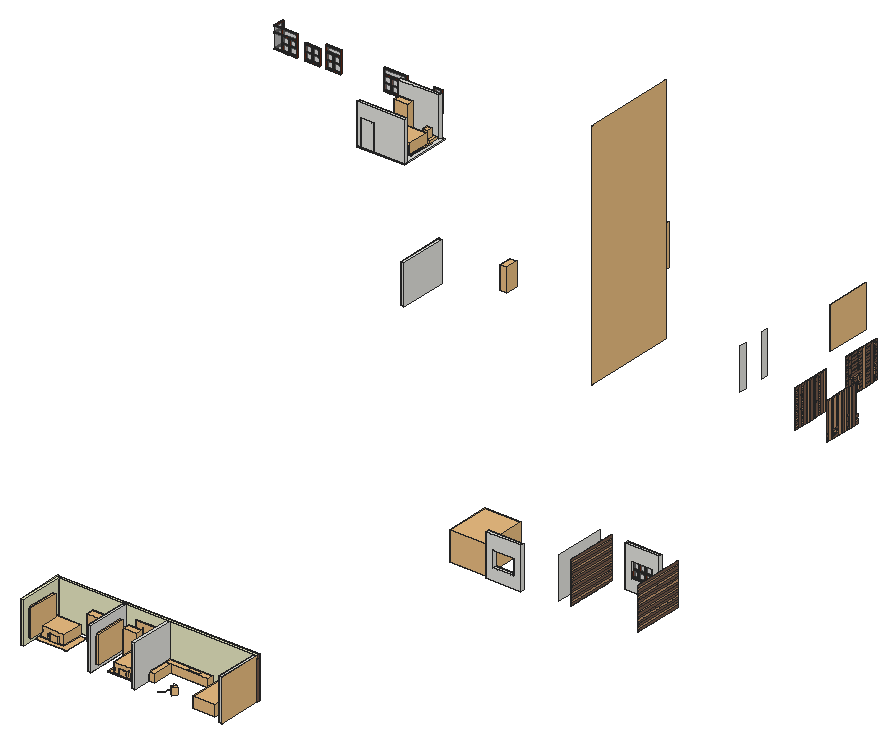
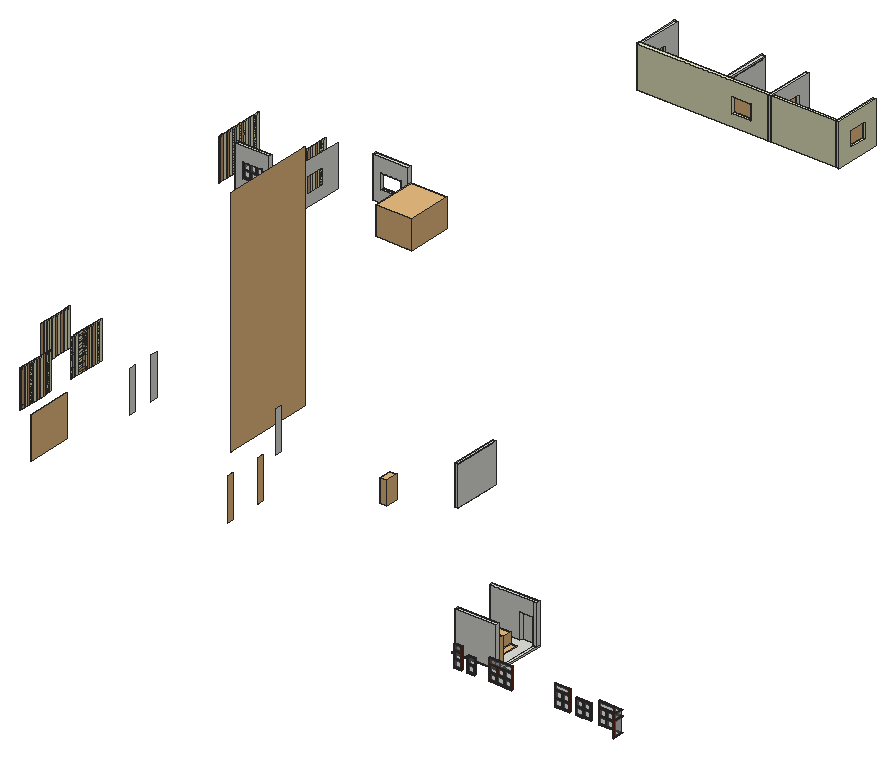
# SketchUp Ruby script. Lengths in inches.
U = 1.inch
M = Sketchup.active_model
def pt(a) = Geom::Point3d.new(a.map { |v| v * U })
def face(e, loops, mat)
  f = e.add_face(loops[0].map { |a| pt(a) })
  loops[1..].each { |l| e.add_face(l.map { |a| pt(a) }).erase! }
  f.material = f.back_material = mat if mat
  f
end
# faces: each face lists its corners as indices into pts; further lists are holes
def faces(e, pts, list, mat = nil) = list.each { |f| face(e, (f[0].is_a?(Array) ? f : [f]).map { |l| l.map { |i| pts[i] } }, mat) }
# xy, xz, yz: faces in a plane at the given z, y or x. An outline is a flat list of corners, or four numbers for a rectangle; further outlines are holes
def ring(l) = l.size == 4 ? [[l[0], l[1]], [l[2], l[1]], [l[2], l[3]], [l[0], l[3]]] : l.each_slice(2).to_a
def flat(e, list, mat, &to3) = list.each { |f| face(e, (f[0].is_a?(Array) ? f : [f]).map { |l| ring(l).map { |u, v| to3.(u, v) } }, mat) }
def xy(e, z, list, mat = nil) = flat(e, list, mat) { |x, y| [x, y, z] }
def xz(e, y, list, mat = nil) = flat(e, list, mat) { |x, z| [x, y, z] }
def yz(e, x, list, mat = nil) = flat(e, list, mat) { |y, z| [x, y, z] }
def lines(e, pts, list) = list.each { |a, b| e.add_line(pt(pts[a]), pt(pts[b])) }
# prism: a flat outline (further loops are holes) pulled along v
def prism(e, loops, v, mat = nil)
  f = face(e, loops, mat); d = Geom::Vector3d.new(v.map { |x| x * U })
  f.pushpull(f.normal.samedirection?(d) ? d.length : -d.length)
end
def box(e, o, s, mat = nil) = prism(e, [[o, [o[0] + s[0], o[1], o[2]], [o[0] + s[0], o[1] + s[1], o[2]], [o[0], o[1] + s[1], o[2]]]], [0, 0, s[2]], mat)
def at(x, y, z, deg = 0) = Geom::Transformation.translation(pt([x, y, z])) * Geom::Transformation.rotation(ORIGIN, Z_AXIS, deg.degrees)
def axes(o, x, y, z) = Geom::Transformation.new([*x, 0, *y, 0, *z, 0, *pt(o).to_a, 1])
def part(name) = M.definitions.add(name)
# library, detail: a bought-in or finely detailed component or shape, given as its bounding box
def library(name, o, s) = part(name).tap { |d| box(d.entities, o, s) }
def detail(e, o, s) = box(e.add_group.entities, o, s)
def put(e, d, t, mat = nil) = e.add_instance(d, t).tap { |i| i.material = mat if mat }
def group(e, t, mat = nil) = e.add_group.tap { |g| g.transformation = t; g.material = mat if mat }.entities
root = M.entities
M.materials.add("02 - Default1").color = [198, 154, 113]
M.materials.add("1").color = [234, 234, 196]
M.materials.add("3").color = [118, 89, 74]
M.materials.add("Material1 metal").color = [192, 192, 192]
M.materials.add("[Color_B17]").color = [102, 40, 20]
M.materials.add("[Translucent_Glass_Gray]").color = [128, 128, 128]
M.materials["[Translucent_Glass_Gray]"].alpha = 0.5
M.materials.add("putih ceramic").color = [255, 255, 255]
c1 = library("HMI+SHE+SAID+BARSTOOL",[-9.1,-9.7,0],[19.23,19.64,34.25])
c2 = part("Component\#33")
prism(c2.entities,[[[0.91,0.01,0.74],[0.87,0.05,0.89],[0.79,0.11,1.01],[0.7,0.18,1.1],[0.58,0.27,1.16],[0.46,0.36,1.18],[0.34,0.46,1.16],[0.23,0.55,1.1],[0.14,0.62,1.01],[0.0625,0.68,0.89],[0.02,0.72,0.74],[0,0.73,0.59],[0.02,0.72,0.4375],[0.0625,0.68,0.3],[0.14,0.62,0.17],[0.23,0.55,0.08],[0.34,0.46,0.02],[0.46,0.36,0],[0.58,0.27,0.02],[0.7,0.18,0.08],[0.79,0.11,0.17],[0.87,0.05,0.3],[0.91,0.01,0.4375],[0.93,0,0.59]]],[0.12,0.15,0],"Material1 metal")
c3 = library("Group10",[-94.75,-3.97,0],[199.87,106.11,39.4375])
c4 = library("mesh-258",[-96.03,-121.28,21.97],[201.42,163.89,40.48])
c5 = library("Group14",[-46.92,-34.29,0],[94.87,68.58,31.875])
c6 = library("Group16",[-47.82,-34.55,0],[96.75,69.58,33.34])
c7 = library("Group18",[-33.62,-26.58,0],[67.24,53.16,20.44])
c8 = library("Group20",[-0.01,-0.01,0.02],[107.76,124.16,6.31])
c9 = library("mesh-263",[-97.08,-118.58,12.75],[201.41,233.93,94.93])
c10 = library("mesh-264",[-106.11,-80.86,12.52],[217.88,74.95,54.44])
c11 = part("Group9")
put(c11.entities,c3,axes([-2.83,3.64,23.125],[0.96274,0,0],[0,0.96274,0],[0,0,0.96274]))
g1 = group(c11.entities,at(-2.83,3.64,23.41))
put(g1,c4,axes([0,0,-21.09],[0.96274,0,0],[0,0.96274,0],[0,0,0.96274]))
put(c11.entities,c5,at(49.15,58.47,50.125))
put(c11.entities,c6,at(-47.3,60.89,49.06))
put(c11.entities,c7,at(-22.74,14.21,61.08))
put(c11.entities,c8,axes([-96.54,-113.26,0],[1.80992,0,0],[0,1.80992,0],[0,0,1.80992]))
g2 = group(c11.entities,at(-2.83,1.61,11.33))
put(g2,c9,at(0,0,-12.75))
g3 = group(c11.entities,at(-2.83,20.36,11.1))
put(g3,c10,at(0,0,-12.52))
c12 = library("Window curtains 2",[0,-81.89,0],[92,82.37,8.12])
c13 = library("Group\#201",[0,0,0],[0.82,117.2,114.11])
c14 = library("mesh-256",[-120.04,-169.59,0.14],[253.19,307.8,1.7])
c15 = part("Group7")
put(c15.entities,c14,at(0,0,0))
c16 = library("COMEDOR+3",[0,0,-3.47],[105.08,67.9,32.46])
c17 = library("Kitchen base cabinets \#1",[0,0,0],[91.73,24.71,35.43])
c18 = library("Group26",[-8.72,-28.73,0.18],[47.65,50.07,77.26])
c19 = library("Group",[-44.49,-44.49,0],[88.98,89.04,25.37])
c20 = library("Dressing_table",[0,-6.3125,-0.01],[54.59,27.125,100.87])
c21 = library("Kitchen base cabinets",[0,0,0],[24.71,188.98,35.43])
c22 = library("coz_ll_125-50",[0,0,0],[49.21,19.69,5.91])
c23 = part("Group\#331")
xy(c23.entities,0,[[0,0,0.82,6.2]],"1")
xy(c23.entities,114.11,[[0,0,0.82,6.2]],"1")
xz(c23.entities,0,[[0,0,0.82,114.11]],"1")
xz(c23.entities,6.2,[[0,0,0.82,114.11]],"1")
yz(c23.entities,0,[[0,0,6.2,114.11]],"1")
yz(c23.entities,0.82,[[0,0,6.2,114.11]],"3")
c24 = part("Group\#330")
put(c24.entities,c23,axes([-0.82,0,0],[1,0,0],[0,1.45243,0],[0,0,1]),"1")
c25 = part("Group\#329")
box(c25.entities,[0,0,0],[0.82,6.2,114.11],"02 - Default1")
c26 = part("Group\#328")
put(c26.entities,c25,axes([-0.82,0,0],[1,0,0],[0,1.45243,0],[0,0,1]))
c27 = part("Group\#286")
put(c27.entities,c24,axes([0.82,0,0],[1,0,0],[0,0.6885,0],[0,0,1]),"02 - Default1")
put(c27.entities,c24,axes([0.82,6.2,89.22],[1,0,0],[0,0,0.67033],[0,-0.05434,0]),"02 - Default1")
put(c27.entities,c24,axes([0.82,6.2,12.68],[1,0,0],[0,0,0.67033],[0,-0.05434,0]),"02 - Default1")
put(c27.entities,c26,axes([0.82,6.2,63.7],[1,0,0],[0,0,0.67033],[0,-0.05434,0]),"02 - Default1")
put(c27.entities,c26,axes([0.82,6.2,25.75],[1,0,0],[0,0,0.67033],[0,-0.05434,0]),"02 - Default1")
put(c27.entities,c26,axes([0.82,6.2,82.99],[1,0,0],[0,0,0.67033],[0,-0.05434,0]),"02 - Default1")
put(c27.entities,c24,axes([0.82,6.2,50.83],[1,0,0],[0,0,0.67033],[0,-0.05434,0]),"02 - Default1")
put(c27.entities,c24,axes([0.82,6.2,76.54],[1,0,0],[0,0,0.67033],[0,-0.05434,0]),"02 - Default1")
put(c27.entities,c24,axes([0.82,6.2,31.98],[1,0,0],[0,0,0.67033],[0,-0.05434,0]),"02 - Default1")
put(c27.entities,c26,axes([0.82,6.2,44.6],[1,0,0],[0,0,0.67033],[0,-0.05434,0]),"02 - Default1")
g4 = group(c27.entities,at(0.82,6.2,95.39),"02 - Default1")
put(g4,c23,axes([-0.82,0,0],[1,0,0],[0,0,0.97361],[0,-0.05434,0]),"1")
put(c27.entities,c26,axes([0.82,6.2,101.84],[1,0,0],[0,0,0.67033],[0,-0.05434,0]),"02 - Default1")
put(c27.entities,c24,axes([0.82,6.2,0],[1,0,0],[0,0,0.67033],[0,-0.05434,0]),"02 - Default1")
put(c27.entities,c24,axes([0.82,6.2,19.3],[1,0,0],[0,0,0.67033],[0,-0.05434,0]),"02 - Default1")
put(c27.entities,c24,axes([0.82,6.2,69.93],[1,0,0],[0,0,0.67033],[0,-0.05434,0]),"02 - Default1")
put(c27.entities,c26,axes([0.82,6.2,6.45],[1,0,0],[0,0,0.67033],[0,-0.05434,0]),"02 - Default1")
put(c27.entities,c24,axes([0.82,6.2,38.15],[1,0,0],[0,0,0.67033],[0,-0.05434,0]),"02 - Default1")
put(c27.entities,c24,axes([0.82,6.2,57.25],[1,0,0],[0,0,0.67033],[0,-0.05434,0]),"02 - Default1")
put(c27.entities,c24,axes([0.82,6.2,108.07],[1,0,0],[0,0,0.67033],[0,-0.05434,0]),"02 - Default1")
c28 = library("kitchen mas haris",[0,0,0],[110.24,135.43,86.61])
c29 = part("Group\#244")
put(c29.entities,c24,axes([0.82,0,0],[1,0,0],[0,0.6885,0],[0,0,1]),"02 - Default1")
put(c29.entities,c26,axes([0.82,6.625,0],[1,0,0],[0,0.6885,0],[0,0,1]),"02 - Default1")
put(c29.entities,c26,axes([0.82,26.45,0],[1,0,0],[0,0.6885,0],[0,0,1]),"02 - Default1")
put(c29.entities,c24,axes([0.82,13.03,0],[1,0,0],[0,0.6885,0],[0,0,1]),"02 - Default1")
put(c29.entities,c24,axes([0.82,32.84,0],[1,0,0],[0,0.6885,0],[0,0,1]),"02 - Default1")
put(c29.entities,c24,axes([0.82,19.82,0],[1,0,0],[0,0.6885,0],[0,0,1]),"02 - Default1")
g5 = group(c29.entities,at(0,117.2,0))
put(g5,c24,axes([0.82,0,0],[1,0,0],[0,0,0.67033],[0,-1.0271,0]),"02 - Default1")
put(g5,c26,axes([0.82,0,101.84],[1,0,0],[0,0,0.67033],[0,-1.0271,0]),"02 - Default1")
put(g5,c26,axes([0.82,0,6.45],[1,0,0],[0,0,0.67033],[0,-1.0271,0]),"02 - Default1")
put(g5,c24,axes([0.82,0,69.93],[1,0,0],[0,0,0.67033],[0,-1.0271,0]),"02 - Default1")
put(g5,c24,axes([0.82,0,95.39],[1,0,0],[0,0,0.67033],[0,-1.0271,0]),"02 - Default1")
put(g5,c24,axes([0.82,0,38.15],[1,0,0],[0,0,0.67033],[0,-1.0271,0]),"02 - Default1")
put(g5,c26,axes([0.82,0,25.75],[1,0,0],[0,0,0.67033],[0,-1.0271,0]),"02 - Default1")
put(g5,c24,axes([0.82,0,31.98],[1,0,0],[0,0,0.67033],[0,-1.0271,0]),"02 - Default1")
put(g5,c24,axes([0.82,0,50.83],[1,0,0],[0,0,0.67033],[0,-1.0271,0]),"02 - Default1")
put(g5,c24,axes([0.82,0,108.07],[1,0,0],[0,0,0.67033],[0,-1.0271,0]),"02 - Default1")
put(g5,c24,axes([0.82,0,89.22],[1,0,0],[0,0,0.67033],[0,-1.0271,0]),"02 - Default1")
put(g5,c24,axes([0.82,0,57.25],[1,0,0],[0,0,0.67033],[0,-1.0271,0]),"02 - Default1")
put(g5,c26,axes([0.82,0,63.7],[1,0,0],[0,0,0.67033],[0,-1.0271,0]),"02 - Default1")
put(g5,c24,axes([0.82,0,12.68],[1,0,0],[0,0,0.67033],[0,-1.0271,0]),"02 - Default1")
put(g5,c26,axes([0.82,0,44.6],[1,0,0],[0,0,0.67033],[0,-1.0271,0]),"02 - Default1")
put(g5,c24,axes([0.82,0,76.54],[1,0,0],[0,0,0.67033],[0,-1.0271,0]),"02 - Default1")
put(g5,c24,axes([0.82,0,19.3],[1,0,0],[0,0,0.67033],[0,-1.0271,0]),"02 - Default1")
put(g5,c26,axes([0.82,0,82.99],[1,0,0],[0,0,0.67033],[0,-1.0271,0]),"02 - Default1")
put(c29.entities,c26,axes([0.82,45.81,0],[1,0,0],[0,0.6885,0],[0,0,1]),"02 - Default1")
put(c29.entities,c24,axes([0.82,52.21,0],[1,0,0],[0,0.6885,0],[0,0,1]),"02 - Default1")
put(c29.entities,c24,axes([0.82,39.18,0],[1,0,0],[0,0.6885,0],[0,0,1]),"02 - Default1")
put(c29.entities,c26,axes([0.82,85.24,0],[1,0,0],[0,0.6885,0],[0,0,1]),"02 - Default1")
put(c29.entities,c24,axes([0.82,78.62,0],[1,0,0],[0,0.6885,0],[0,0,1]),"02 - Default1")
put(c29.entities,c24,axes([0.82,58.8,0],[1,0,0],[0,0.6885,0],[0,0,1]),"02 - Default1")
put(c29.entities,c26,axes([0.82,65.42,0],[1,0,0],[0,0.6885,0],[0,0,1]),"02 - Default1")
put(c29.entities,c24,axes([0.82,71.82,0],[1,0,0],[0,0.6885,0],[0,0,1]),"02 - Default1")
put(c29.entities,c24,axes([0.82,91.64,0],[1,0,0],[0,0.6885,0],[0,0,1]),"02 - Default1")
put(c29.entities,c26,axes([0.82,104.6,0],[1,0,0],[0,0.6885,0],[0,0,1]),"02 - Default1")
put(c29.entities,c24,axes([0.82,111,0],[1,0,0],[0,0.6885,0],[0,0,1]),"02 - Default1")
put(c29.entities,c24,axes([0.82,97.98,0],[1,0,0],[0,0.6885,0],[0,0,1]),"02 - Default1")
c30 = part("Framed panel")
g6 = group(c30.entities,at(0,0,0))
prism(g6,[[[0,22.64,0],[21.26,22.64,0],[21.26,0,0],[0,0,0]],[[1.57,1.57,0],[19.69,1.57,0],[19.69,21.0625,0],[1.57,21.0625,0]]],[0,0,1.57],"[Color_B17]")
g7 = group(c30.entities,at(1.57,1.57,1.02))
xy(g7,0,[[0,0,18.11,19.49]],"[Translucent_Glass_Gray]")
c31 = part("Group\#25")
put(c31.entities,c30,at(0,21.0625,1.57))
put(c31.entities,c30,at(0,0,0))
c32 = part("Group\#47")
g8 = group(c32.entities,at(0,0,0))
prism(g8,[[[70.87,0,0],[0,0,0],[0,47.24,0],[70.87,47.24,0]],[[47.83,1.77,0],[69.09,1.77,0],[69.09,45.47,0],[47.83,45.47,0]],[[46.0625,45.47,0],[24.8,45.47,0],[24.8,1.77,0],[46.0625,1.77,0]],[[1.77,1.77,0],[23.03,1.77,0],[23.03,45.47,0],[1.77,45.47,0]]],[0,0,4.33],"[Color_B17]")
put(c32.entities,c31,at(1.77,1.77,0.59))
put(c32.entities,c31,at(24.8,1.77,0.59))
put(c32.entities,c31,at(47.83,1.77,0.59))
c33 = part("Group\#94")
xz(c33.entities,0,[[0,0,144,120]])
g9 = group(c33.entities,at(0,0,0))
yz(g9,0,[[0,0,10,120]])
p = [[0,0,120],[134,0,120],[134,0,0],[0,0,0]]
lines(g9,p,[[0,1],[2,3]])
g10 = group(g9,at(0,0,0))
xy(g10,0,[[0,0,144,10]])
xy(g10,120,[[0,0,144,10]])
xz(g10,10,[[0,0,144,120]])
yz(g10,144,[[0,0,10,120]])
c34 = library("cnc-jali.dxf",[0,0,0],[286,708,0.01])
c35 = part("Group\#91")
yz(c35.entities,0,[[0,0,19.46,126.79]])
c36 = library("Group\#10",[0,0,0],[37.44,20.12,70.98])
c37 = library("Group\#223",[0,0,0],[5,19.46,126.79])
c38 = library("Group\#212",[0,0,0],[5,19.46,126.79])
c39 = library("Group\#203",[0,0,0],[0.82,117.2,114.11])
c40 = part("DOOR12")
g11 = group(c40.entities,at(114.73,28.14,-0.51))
g12 = group(g11,at(0,0,0))
box(g12,[0,0,0],[36,0.5,77.7])
c41 = part("Group\#193")
prism(c41.entities,[[[0,134,120],[0,134,0],[0,41,0],[0,41,78],[0,2,78],[0,2,0],[0,-10,0],[0,-10,120]]],[10,0,0])
c42 = part("Window Frame 001")
prism(c42.entities,[[[0,22.64,0],[20.08,22.64,0],[20.08,0,0],[0,0,0]],[[1.57,1.57,0],[18.5,1.57,0],[18.5,21.0625,0],[1.57,21.0625,0]]],[0,0,1.57],"[Color_B17]")
c43 = part("Group\#14")
put(c43.entities,c42,at(0,0,0))
g13 = group(c43.entities,at(1.57,1.57,1.02))
xy(g13,0,[[0,0,16.93,19.49]],"[Translucent_Glass_Gray]")
c44 = part("Group\#21")
put(c44.entities,c43,at(0,21.0625,1.57))
put(c44.entities,c43,at(0,0,0))
c45 = part("Group\#23")
xy(c45.entities,0,[[0,0,67.32,15.94]],"[Translucent_Glass_Gray]")
c46 = part("Window Frame 004")
prism(c46.entities,[[[20.96,22.64,0],[20.96,0,0],[0,0,0],[0,22.64,0]],[[19.39,21.0625,0],[1.57,21.0625,0],[1.57,1.57,0],[19.39,1.57,0]]],[0,0,1.57],"[Color_B17]")
c47 = part("Group\#20")
put(c47.entities,c46,at(0,0,0))
g14 = group(c47.entities,at(1.57,1.57,1.02))
xy(g14,0,[[0,0,17.81,19.49]],"[Translucent_Glass_Gray]")
c48 = part("Group\#28")
put(c48.entities,c47,at(0,21.0625,1.57))
put(c48.entities,c47,at(0,0,0))
c49 = part("Group\#35")
xz(c49.entities,0,[[0,0,44.29,15.94]],"[Translucent_Glass_Gray]")
xy(root,0,[[1932.8125,380.85,1942.8125,514.85],[1992.71,1328.88,2098.97,1338.88]])
xy(root,2.72,[[1732.17,402.25,1731.85,402.51,1757.375,434.99,1757.69,434.74]],"putih ceramic")
xy(root,3.26,[[1732.17,402.25,1757.69,434.74,1757.375,434.99,1731.97,402.66,1731.85,402.51]],"putih ceramic")
xy(root,36,[[1932.8125,427.84,1942.8125,489.84],[2014.04,1328.88,2076.72,1338.88]])
xy(root,84,[[1932.8125,427.84,1942.8125,489.84],[2014.04,1328.88,2076.72,1338.88]])
xy(root,126.79,[[1932.8125,380.85,1942.8125,514.85],[1992.71,1328.88,2098.97,1338.88]])
xz(root,380.85,[[1932.8125,0,1942.8125,126.79]])
xz(root,427.84,[[1932.8125,36,1942.8125,84]])
xz(root,489.84,[[1932.8125,36,1942.8125,84]])
xz(root,514.85,[[1932.8125,0,1942.8125,126.79]])
xz(root,1328.88,[[[1992.71,0,2098.97,126.79],[2014.04,36,2076.72,84]]])
xz(root,1338.88,[[[1992.71,0,2098.97,126.79],[2014.04,36,2076.72,84]]])
yz(root,1932.8125,[[[380.85,0,514.85,126.79],[427.84,36,489.84,84]]])
yz(root,1942.8125,[[[380.85,0,514.85,126.79],[427.84,36,489.84,84]]])
yz(root,1992.71,[[1328.88,0,1338.88,126.79]])
yz(root,2014.04,[[1328.88,36,1338.88,84]])
yz(root,2076.72,[[1328.88,36,1338.88,84]])
yz(root,2098.97,[[1328.88,0,1338.88,126.79]])
p = [[1757.69,434.74,2.72],[1757.69,434.74,3.26],[1732.17,402.25,3.26],[1732.17,402.25,2.72],[1757.375,434.99,3.26],[1757.375,434.99,2.72],
  [1731.85,402.51,2.72],[1731.85,402.51,3.26],[1731.97,402.66,3.26],[445.36,2937.05,0],[445.36,2793.05,0],[445.36,2793.05,120],
  [1543.51,524.85,0],[1543.51,380.85,0]]
faces(root,p,[[0,1,2,3],[4,5,6,7,8],[5,4,1,0]],"putih ceramic")
lines(root,p,[[9,10],[10,11],[12,13]])
put(root,c1,axes([1764.51,422.42,0],[-0.54256,0.4263,0],[-0.4263,-0.54256,0],[0,0,0.5865]))
put(root,c2,axes([1755.57,432.9,5.7],[0,-0.69,0],[0.69,0,0],[0,0,0.69]))
put(root,c2,axes([1755.57,432.9,19.56],[0,-0.69,0],[0.69,0,0],[0,0,0.69]))
put(root,c11,axes([1626.26,442.625,0.07],[0,-0.31173,0],[0.31173,0,0],[0,0,0.31173]))
put(root,c12,axes([1337.47,400.2,97.04],[0,1,0],[0,0,1],[1,0,0]))
put(root,c12,axes([1543.51,400.2,97.04],[0,1,0],[0,0,1],[1,0,0]))
put(root,c13,axes([1942.8125,380.85,0],[1,0,0],[0,1.14,0],[0,0,1.11]))
g15 = group(root,at(1667.51,514.85,0))
yz(g15,0,[[-134,0,0,120]])
g16 = group(g15,at(0,0,0))
xz(g16,0,[[0,0,10,120]])
p = [[0,0,120],[0,-124.69,120],[0,-124.69,0],[0,0,0]]
lines(g16,p,[[0,1],[2,3]])
g17 = group(g16,at(0,0,0))
xy(g17,0,[[0,-134,10,0]])
xy(g17,126.79,[[0,-134,10,0]])
xz(g17,-134,[[0,0,10,126.79]])
yz(g17,10,[[-134,0,0,126.79]])
put(root,c15,axes([1624.43,450.87,-0.02],[0,-0.31173,0],[0.31173,0,0],[0,0,0.31173]))
put(root,c16,at(1909.65,397.43,3.47,90))
g18 = group(root,at(1533.51,524.85,0,-90))
xy(g18,0,[[0,0,144,10]])
xy(g18,36,[[46,0,108,10]])
xy(g18,84,[[46,0,108,10]])
xy(g18,126.79,[[0,0,144,10]])
xz(g18,0,[[[0,0,144,126.79],[46,36,108,84]]])
xz(g18,10,[[[0,0,144,126.79],[46,36,108,84]]])
yz(g18,0,[[0,0,10,126.79]])
yz(g18,46,[[0,36,10,84]])
yz(g18,108,[[0,36,10,84]])
yz(g18,144,[[0,0,10,126.79]])
g19 = group(root,at(1327.47,524.85,0),"1")
xy(g19,0,[[0,-144,10,0]])
xy(g19,36,[[0,-104.81,10,-44.64]])
xy(g19,84,[[0,-104.81,10,-44.64]])
xy(g19,126.79,[[0,-144,10,0]])
xz(g19,-144,[[0,0,10,126.79]])
xz(g19,-104.81,[[0,36,10,84]])
xz(g19,-44.64,[[0,36,10,84]])
xz(g19,0,[[0,0,10,126.79]])
yz(g19,0,[[[-144,0,0,126.79],[-104.81,36,-44.64,84]]])
yz(g19,10,[[[-144,0,0,126.79],[-104.81,36,-44.64,84]]])
put(root,c15,axes([1380.56,461.81,-0.02],[0,0.31173,0],[-0.31173,0,0],[0,0,0.31173]))
put(root,c17,axes([1677.51,498.55,0],[0,-0.69,0],[0.69,0,0],[0,0,0.69]))
put(root,c11,axes([1378.72,470.06,0.07],[0,0.31173,0],[-0.31173,0,0],[0,0,0.31173]))
put(root,c18,axes([1649.92,499.91,7.53],[0,-0.31173,0],[0.31173,0,0],[0,0,0.31173]))
put(root,c19,axes([1650.52,498.91,0],[-0.31114,0.01926,0],[-0.01926,-0.31114,0],[0,0,0.31173]))
put(root,c20,axes([1552.89,496.6,0.01],[0.75,0,0],[0,0.75,0],[0,0,0.75]))
put(root,c20,axes([1440.87,499.24,0.01],[0.75,0,0],[0,0.75,0],[0,0,0.75]))
put(root,c21,axes([1677.51,514.85,0],[0,-0.69,0],[0.69,0,0],[0,0,0.69]))
put(root,c22,axes([1743.25,499.63,20.52],[0.69,0,0],[0,0.69,0],[0,0,0.69]))
put(root,c12,axes([1575.51,514.85,97.04],[1,0,0],[0,0,1],[0,-0.16,0]))
put(root,c27,axes([1942.8125,514.9375,0],[1,0,0],[0,1,0],[0,0,1.11]))
g20 = group(root,at(1677.51,524.85,0,180),"1")
xy(g20,0,[[-265.31,0,340.04,10]])
xy(g20,36,[[22.25,0,82.48,10]])
xy(g20,84,[[22.25,0,82.48,10]])
xy(g20,126.79,[[-265.31,0,340.04,10]])
xz(g20,0,[[[-265.31,0,340.04,126.79],[22.25,36,82.48,84]]])
xz(g20,10,[[[-265.31,0,340.04,126.79],[22.25,36,82.48,84]]])
yz(g20,-265.31,[[0,0,10,126.79]])
yz(g20,22.25,[[0,36,10,84]])
yz(g20,82.48,[[0,36,10,84]])
yz(g20,340.04,[[0,0,10,126.79]])
put(root,c27,axes([1942.8125,521.14,0.13],[1,0,0],[0,0.59904,0],[0,0,1.11]))
put(root,c28,at(1873.91,1336.96,0))
put(root,c29,axes([2438.97,1348.92,0],[1,0,0],[0,1.31396,0],[0,0,1.11111]))
put(root,c29,axes([2235.51,1348.92,0],[1,0,0],[0,1.31396,0],[0,0,1.11111]))
g21 = group(root,at(2199.54,1348.92,0))
g22 = group(g21,at(0,0,0))
yz(g22,0,[[[0,0,154,126.79],[56.99,36,118.99,84]]])
g23 = group(root,at(2285.45,1492.92,0))
xy(g23,0,[[0,0,103.96,10]])
xy(g23,36,[[21.49,0,81.72,10]])
xy(g23,84,[[21.49,0,81.72,10]])
xy(g23,126.79,[[0,0,103.96,10]])
xz(g23,0,[[[0,0,103.96,126.79],[21.49,36,81.72,84]]])
xz(g23,10,[[[0,0,103.96,126.79],[21.49,36,81.72,84]]])
yz(g23,0,[[0,0,10,126.79]])
yz(g23,21.49,[[0,36,10,84]])
yz(g23,81.72,[[0,36,10,84]])
yz(g23,103.96,[[0,0,10,126.79]])
put(g23,c32,axes([81.0625,3.375,36],[-0.87489,0,0],[0,0,1.016],[0,1,0]))
put(root,c33,at(1004.02,2382.6875,0,-90))
put(root,c24,axes([2215.32,2353.04,0],[1,0,0],[0,0.6885,0],[0,0,1]),"02 - Default1")
put(root,c26,axes([2215.32,2359.67,0],[1,0,0],[0,0.6885,0],[0,0,1]),"02 - Default1")
put(root,c34,axes([1600.21,2507.64,0],[0,-1,0],[0,0,1],[-1,0,0]))
put(root,c24,axes([2215.32,2366.07,0],[1,0,0],[0,0.6885,0],[0,0,1]),"02 - Default1")
put(root,c24,axes([2215.32,2372.86,0],[1,0,0],[0,0.6885,0],[0,0,1]),"02 - Default1")
put(root,c26,axes([2215.32,2379.49,0],[1,0,0],[0,0.6885,0],[0,0,1]),"02 - Default1")
put(root,c24,axes([2215.32,2385.89,0],[1,0,0],[0,0.6885,0],[0,0,1]),"02 - Default1")
put(root,c24,axes([2215.32,2392.22,0],[1,0,0],[0,0.6885,0],[0,0,1]),"02 - Default1")
put(root,c26,axes([2215.32,2398.85,0],[1,0,0],[0,0.6885,0],[0,0,1]),"02 - Default1")
put(root,c24,axes([2215.32,2405.25,0],[1,0,0],[0,0.6885,0],[0,0,1]),"02 - Default1")
put(root,c29,at(2117.54,2353.04,0))
put(root,c24,axes([2215.32,2470.24,0],[1,0,0],[0,0,0.67033],[0,-1.0271,0]),"02 - Default1")
put(root,c26,axes([2215.32,2470.24,6.45],[1,0,0],[0,0,0.67033],[0,-1.0271,0]),"02 - Default1")
put(root,c24,axes([2215.32,2470.24,19.3],[1,0,0],[0,0,0.67033],[0,-1.0271,0]),"02 - Default1")
put(root,c24,axes([2215.32,2411.84,0],[1,0,0],[0,0.6885,0],[0,0,1]),"02 - Default1")
put(root,c26,axes([2215.32,2418.46,0],[1,0,0],[0,0.6885,0],[0,0,1]),"02 - Default1")
put(root,c35,at(1900.15,2415.34,0))
put(root,c24,axes([2215.32,2424.86,0],[1,0,0],[0,0.6885,0],[0,0,1]),"02 - Default1")
put(root,c24,axes([2215.32,2431.66,0],[1,0,0],[0,0.6885,0],[0,0,1]),"02 - Default1")
put(root,c26,axes([2215.32,2438.28,0],[1,0,0],[0,0.6885,0],[0,0,1]),"02 - Default1")
put(root,c35,at(1505.21,2432.92,0))
put(root,c24,axes([2215.32,2444.68,0],[1,0,0],[0,0.6885,0],[0,0,1]),"02 - Default1")
put(root,c24,axes([2215.32,2451.02,0],[1,0,0],[0,0.6885,0],[0,0,1]),"02 - Default1")
put(root,c25,at(2214.49,2457.64,0),"02 - Default1")
put(root,c36,axes([1163.93,2481.26,0],[0,-1,0],[-1,0,0],[0,0,1]))
put(root,c35,at(1900.15,2498.56,0))
put(root,c29,at(2117.54,2545.15,0))
put(root,c37,axes([1389.45,2647.39,0],[0.12,0,0],[0,1,0],[0,0,1]))
put(root,c38,axes([1389.4,2761.9375,0],[0.13,0,0],[0,1,0],[0,0,1]))
put(root,c39,axes([1942.8125,2705.65,0.13],[1,0,0],[0,1.14,0],[0,0,1.11]))
put(root,c40,axes([323.07,2754.91,0.51],[1.08333,0,0],[0,1,0],[0,0,1]))
put(root,c41,at(445.36,2793.05,0,-90))
put(root,c11,axes([528.11,2854.82,0.07],[0,-0.31173,0],[0.31173,0,0],[0,0,0.31173]))
g24 = group(root,at(435.36,2937.05,-4,-90))
box(g24,[0,0,0],[154,144,4])
put(root,c15,axes([526.28,2863.07,-0.02],[0,-0.31173,0],[0.31173,0,0],[0,0,0.31173]))
put(root,c18,axes([551.77,2912.11,7.53],[0,-0.31173,0],[0.31173,0,0],[0,0,0.31173]))
put(root,c19,axes([552.37,2911.1,0],[-0.31114,0.01926,0],[-0.01926,-0.31114,0],[0,0,0.31173]))
put(root,c20,axes([448.84,2911.44,0.01],[0.75,0,0],[0,0.75,0],[0,0,0.75]))
g25 = group(root,at(445.36,2937.05,0,-90))
xz(g25,0,[[0,0,10,120]])
g26 = group(g25,at(0,0,0))
xy(g26,0,[[0,0,10,124]])
xy(g26,120,[[0,0,10,124]])
xz(g26,124,[[0,0,10,120]])
yz(g26,0,[[0,0,124,120]])
yz(g26,10,[[0,0,124,120]])
g27 = group(root,at(489.26,3013.2,12.76))
g28 = group(g27,at(1.77,-2.76,47.24))
xz(g28,0,[[0,0,20.08,15.94]],"[Translucent_Glass_Gray]")
g29 = group(g27,at(0,0,0))
prism(g29,[[[0,0,64.96],[23.62,0,64.96],[23.62,0,0],[0,0,0]],[[21.85,0,1.77],[21.85,0,45.47],[1.77,0,45.47],[1.77,0,1.77]],[[1.77,0,47.24],[21.85,0,47.24],[21.85,0,63.1875],[1.77,0,63.1875]]],[0,-4.33,0],"[Color_B17]")
put(g27,c44,axes([1.77,-0.59,1.77],[1,0,0],[0,0,1],[0,-1,0]))
g30 = group(root,at(447.98,3013.2,12.76))
g31 = group(g30,at(0,0,0))
prism(g31,[[[0,0,47.24],[23.62,0,47.24],[23.62,0,0],[0,0,0]],[[21.85,0,1.77],[21.85,0,45.47],[1.77,0,45.47],[1.77,0,1.77]]],[0,-4.33,0],"[Color_B17]")
put(g30,c44,axes([1.77,-0.59,1.77],[1,0,0],[0,0,1],[0,-1,0]))
g32 = group(root,at(334.5,3013.2,12.76))
put(g32,c31,axes([1.77,-0.59,1.77],[1,0,0],[0,0,1],[0,-1,0]))
put(g32,c31,axes([24.8,-0.59,1.77],[1,0,0],[0,0,1],[0,-1,0]))
put(g32,c31,axes([47.83,-0.59,1.77],[1,0,0],[0,0,1],[0,-1,0]))
g33 = group(g32,at(0,0,0))
prism(g33,[[[0,0,64.96],[70.87,0,64.96],[70.87,0,0],[0,0,0]],[[1.77,0,47.24],[69.09,0,47.24],[69.09,0,63.1875],[1.77,0,63.1875]],[[47.83,0,1.77],[69.09,0,1.77],[69.09,0,45.47],[47.83,0,45.47]],[[46.0625,0,45.47],[24.8,0,45.47],[24.8,0,1.77],[46.0625,0,1.77]],[[1.77,0,1.77],[23.03,0,1.77],[23.03,0,45.47],[1.77,0,45.47]]],[0,-4.33,0],"[Color_B17]")
put(g32,c45,axes([1.77,-2.76,47.24],[1,0,0],[0,0,1],[0,-1,0]))
g34 = group(root,at(158.29,3013.2,12.76))
g35 = group(g34,at(0,0,0))
prism(g35,[[[0,0,64.96],[47.24,0,64.96],[47.24,0,0],[0,0,0]],[[45.47,0,45.47],[24.51,0,45.47],[24.51,0,1.77],[45.47,0,1.77]],[[22.74,0,45.47],[1.77,0,45.47],[1.77,0,1.77],[22.74,0,1.77]],[[1.77,0,47.24],[45.47,0,47.24],[45.47,0,63.1875],[1.77,0,63.1875]]],[0,-4.33,0],"[Color_B17]")
put(g34,c48,axes([1.77,-0.59,1.77],[1,0,0],[0,0,1],[0,-1,0]))
put(g34,c48,axes([24.51,-0.59,1.77],[1,0,0],[0,0,1],[0,-1,0]))
g36 = group(g34,at(1.77,-2.76,47.24))
xz(g36,0,[[0,0,43.7,15.94]],"[Translucent_Glass_Gray]")
g37 = group(root,at(94.08,3013.2,12.76))
g38 = group(g37,at(0,0,0))
prism(g38,[[[0,0,47.24],[47.24,0,47.24],[47.24,0,0],[0,0,0]],[[45.47,0,45.47],[24.51,0,45.47],[24.51,0,1.77],[45.47,0,1.77]],[[22.74,0,45.47],[1.77,0,45.47],[1.77,0,1.77],[22.74,0,1.77]]],[0,-4.33,0],"[Color_B17]")
put(g37,c48,axes([1.77,-0.59,1.77],[1,0,0],[0,0,1],[0,-1,0]))
put(g37,c48,axes([24.51,-0.59,1.77],[1,0,0],[0,0,1],[0,-1,0]))
g39 = group(root,at(0,3008.3,10.95))
put(g39,c31,axes([48.53,0.59,45.47],[1,0,0],[0,0,-1],[0,1,0]))
put(g39,c31,axes([25.49,0.59,45.47],[1,0,0],[0,0,-1],[0,1,0]))
put(g39,c49,at(25.49,1.57,47.25))
g40 = group(g39,at(1.57,1.57,1.77))
xz(g40,0,[[0,0,22.15,43.7]],"[Translucent_Glass_Gray]")
yz(g40,0,[[0,0,29.92,43.7]],"[Translucent_Glass_Gray]")
p = [[22.15,2.76,0],[22.15,0,0],[22.15,2.76,43.7],[22.15,0,43.7],[2.76,2.76,43.7],[2.76,29.92,43.7],
  [0,29.92,43.7],[0,29.92,0],[2.76,29.92,0],[2.76,2.76,0]]
lines(g40,p,[[0,1],[0,2],[2,3],[4,2],[5,4],[6,5],[7,8],[8,5],[8,9],[9,0]])
g41 = group(g39,at(0,0,0))
xy(g41,0,[[0,0,0,33.27,4.33,33.27,4.33,4.33,71.56,4.33,71.56,0]],"[Color_B17]")
xy(g41,1.77,[[0,0,23.72,0,23.72,4.33,4.33,4.33,4.33,31.5,0,31.5],[25.49,0,46.75,4.33],[48.53,0,69.79,4.33]],"[Color_B17]")
xy(g41,45.47,[[0,0,0,31.5,4.33,31.5,4.33,4.33,23.72,4.33,23.72,0],[25.49,0,46.75,4.33],[48.53,0,69.79,4.33]],"[Color_B17]")
xy(g41,47.25,[[0,0,23.72,0,23.72,4.33,4.33,4.33,4.33,31.5,0,31.5],[25.49,0,69.79,4.33]],"[Color_B17]")
xy(g41,63.1875,[[0,0,0,31.5,4.33,31.5,4.33,4.33,23.72,4.33,23.72,0],[25.49,0,69.79,4.33]],"[Color_B17]")
xy(g41,64.96,[[0,0,71.56,0,71.56,4.33,4.33,4.33,4.33,33.27,0,33.27]],"[Color_B17]")
xz(g41,0,[[[0,0,71.56,0,71.56,64.96,0,64.96,0,63.1875,23.72,63.1875,23.72,47.25,0,47.25,0,45.47,23.72,45.47,23.72,1.77,0,1.77],[25.49,1.77,46.75,45.47],[48.53,1.77,69.79,45.47],[25.49,47.25,69.79,63.1875]]],"[Color_B17]")
xz(g41,4.33,[[[4.33,0,4.33,1.77,23.72,1.77,23.72,45.47,4.33,45.47,4.33,47.25,23.72,47.25,23.72,63.1875,4.33,63.1875,4.33,64.96,71.56,64.96,71.56,0],[25.49,1.77,46.75,45.47],[48.53,1.77,69.79,45.47],[25.49,47.25,69.79,63.1875]]],"[Color_B17]")
xz(g41,31.5,[[0,1.77,4.33,45.47],[0,47.25,4.33,63.1875]],"[Color_B17]")
xz(g41,33.27,[[0,0,4.33,64.96]],"[Color_B17]")
yz(g41,0,[[0,0,0,1.77,31.5,1.77,31.5,45.47,0,45.47,0,47.25,31.5,47.25,31.5,63.1875,0,63.1875,0,64.96,33.27,64.96,33.27,0]],"[Color_B17]")
yz(g41,4.33,[[4.33,0,33.27,0,33.27,64.96,4.33,64.96,4.33,63.1875,31.5,63.1875,31.5,47.25,4.33,47.25,4.33,45.47,31.5,45.47,31.5,1.77,4.33,1.77]],"[Color_B17]")
yz(g41,23.72,[[0,1.77,4.33,45.47],[0,47.25,4.33,63.1875]],"[Color_B17]")
yz(g41,25.49,[[0,1.77,4.33,45.47],[0,47.25,4.33,63.1875]],"[Color_B17]")
yz(g41,46.75,[[0,1.77,4.33,45.47]],"[Color_B17]")
yz(g41,48.53,[[0,1.77,4.33,45.47]],"[Color_B17]")
yz(g41,69.79,[[0,1.77,4.33,45.47],[0,47.25,4.33,63.1875]],"[Color_B17]")
yz(g41,71.56,[[0,0,4.33,64.96]],"[Color_B17]")
g42 = group(g39,at(1.57,1.57,47.25))
xz(g42,0,[[0,0,22.15,15.94]],"[Translucent_Glass_Gray]")
yz(g42,0,[[0,0,29.92,15.94]],"[Translucent_Glass_Gray]")
